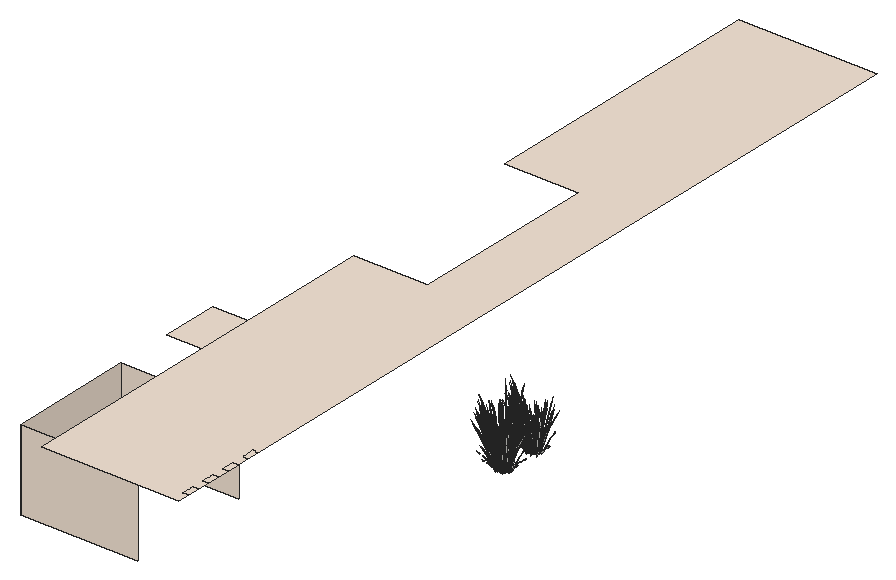
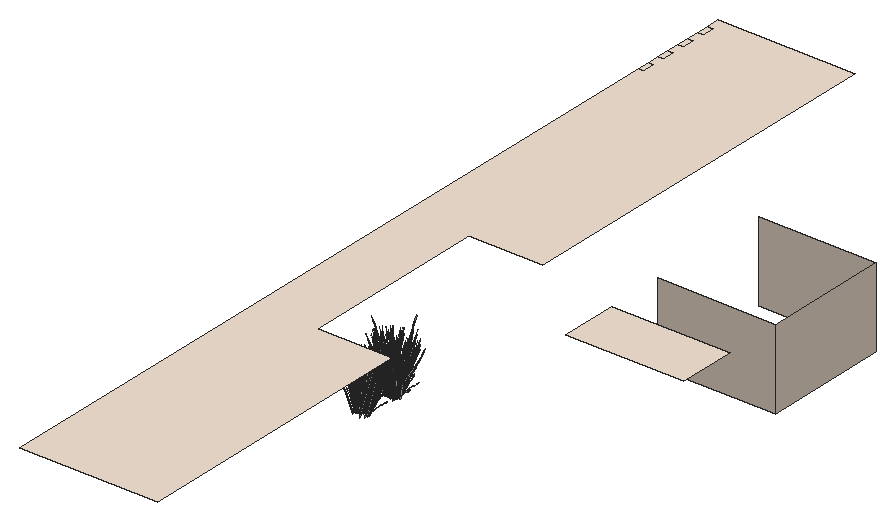
# SketchUp Ruby script. Lengths in inches.
U = 1.inch
M = Sketchup.active_model
def pt(a) = Geom::Point3d.new(a.map { |v| v * U })
def face(e, loops, mat)
  f = e.add_face(loops[0].map { |a| pt(a) })
  loops[1..].each { |l| e.add_face(l.map { |a| pt(a) }).erase! }
  f.material = f.back_material = mat if mat
  f
end
# faces: each face lists its corners as indices into pts; further lists are holes
def faces(e, pts, list, mat = nil) = list.each { |f| face(e, (f[0].is_a?(Array) ? f : [f]).map { |l| l.map { |i| pts[i] } }, mat) }
# xy, xz, yz: faces in a plane at the given z, y or x. An outline is a flat list of corners, or four numbers for a rectangle; further outlines are holes
def ring(l) = l.size == 4 ? [[l[0], l[1]], [l[2], l[1]], [l[2], l[3]], [l[0], l[3]]] : l.each_slice(2).to_a
def flat(e, list, mat, &to3) = list.each { |f| face(e, (f[0].is_a?(Array) ? f : [f]).map { |l| ring(l).map { |u, v| to3.(u, v) } }, mat) }
def xy(e, z, list, mat = nil) = flat(e, list, mat) { |x, y| [x, y, z] }
def xz(e, y, list, mat = nil) = flat(e, list, mat) { |x, z| [x, y, z] }
def yz(e, x, list, mat = nil) = flat(e, list, mat) { |y, z| [x, y, z] }
def lines(e, pts, list) = list.each { |a, b| e.add_line(pt(pts[a]), pt(pts[b])) }
# prism: a flat outline (further loops are holes) pulled along v
def prism(e, loops, v, mat = nil)
  f = face(e, loops, mat); d = Geom::Vector3d.new(v.map { |x| x * U })
  f.pushpull(f.normal.samedirection?(d) ? d.length : -d.length)
end
def box(e, o, s, mat = nil) = prism(e, [[o, [o[0] + s[0], o[1], o[2]], [o[0] + s[0], o[1] + s[1], o[2]], [o[0], o[1] + s[1], o[2]]]], [0, 0, s[2]], mat)
def at(x, y, z, deg = 0) = Geom::Transformation.translation(pt([x, y, z])) * Geom::Transformation.rotation(ORIGIN, Z_AXIS, deg.degrees)
def axes(o, x, y, z) = Geom::Transformation.new([*x, 0, *y, 0, *z, 0, *pt(o).to_a, 1])
def part(name) = M.definitions.add(name)
# library, detail: a bought-in or finely detailed component or shape, given as its bounding box
def library(name, o, s) = part(name).tap { |d| box(d.entities, o, s) }
def detail(e, o, s) = box(e.add_group.entities, o, s)
def put(e, d, t, mat = nil) = e.add_instance(d, t).tap { |i| i.material = mat if mat }
def group(e, t, mat = nil) = e.add_group.tap { |g| g.transformation = t; g.material = mat if mat }.entities
root = M.entities
M.materials.add("C01_Vanilla_Cream").color = [244, 228, 212]
M.materials.add("LightPink_Translucent").color = [144, 107, 117]
M.materials["LightPink_Translucent"].alpha = 0.75
c1 = part("blade")
p = [[2.15,0.21,22],[0,0.17,0],[0.09,0.45,0],[2.18,0.31,22],[2.29,0.31,22],[0.38,0.45,0],
  [2.48,0.24,33],[2.49,0.24,33],[2.48,0.22,33]]
faces(c1.entities,p,[[0,1,2,3],[4,5,2,3],[6,3,4,7],[8,0,3,6]])
c2 = part("seeds")
p = [[0.3,-0.1,1.38],[-0.01,-0.03,1.59],[-0.01,-0.03,0.03],[0.14,-0.07,-0.07],[0.29,-0.03,3],[0.15,0.01,3.11]]
faces(c2.entities,p,[[0,1,2,3],[1,0,4,5]],"LightPink_Translucent")
c3 = part("blade with seeds")
put(c3.entities,c1,at(0,0,0))
put(c3.entities,c2,axes([2.4,0.25,30.99],[1.5799,-0.05474,1.17369],[-0.12525,1.92788,0.29478],[-0.07173,-0.02425,1.56792]))
xy(root,393,[[226.53,171,288,201]],"C01_Vanilla_Cream")
xy(root,432,[[288,12,288,216,326.85,216,326.85,314.71,288,314.71,288,468,360,468,360,63.65,357,63.65,357,57.2,360,57.2,360,50.74,357,50.74,357,44.28,360,44.28,360,37.83,357,37.83,357,31.37,360,31.37,360,24.91,357,24.91,357,18.46,360,18.46,360,12],[357,18.46,360,24.91],[357,31.37,360,37.83],[357,44.28,360,50.74],[357,57.2,360,63.65]],"C01_Vanilla_Cream")
xz(root,75,[[226.53,351,288,393]],"C01_Vanilla_Cream")
xz(root,141,[[226.53,351,288,393]],"C01_Vanilla_Cream")
yz(root,226.53,[[75,351,141,393]],"C01_Vanilla_Cream")
put(root,c3,axes([356.25,225,350.91],[0.12726,0.15818,1.28532],[-0.58807,0.13317,0.10393],[-0.13291,-0.24832,0.54946]))
put(root,c3,axes([357.22,223.95,351.54],[-0.08515,-0.06907,1.31208],[-0.56828,0.04379,-0.2075],[-0.0907,-0.16522,0.10523]))
put(root,c3,axes([357.82,225.12,351.74],[-0.26572,-0.40059,-0.53284],[0.54698,-0.22325,0.0643],[-0.06214,-0.19355,0.75375]))
put(root,c3,axes([358.92,225.51,351.74],[0.01449,-0.45571,-0.53284],[0.61002,0.03061,0.0643],[0.06438,-0.19306,0.75375]))
put(root,c3,axes([359.77,224.8,351.54],[-0.00537,-0.09805,1.31208],[-0.45391,-0.28338,-0.2075],[0.07018,-0.17178,0.10523]))
put(root,c3,axes([357.87,224.78,351.39],[0.16784,-0.37886,-0.2656],[0.48968,0.1105,0.3429],[-0.0449,-0.15254,0.65611]))
put(root,c3,axes([358.24,225.28,350.91],[-0.10366,0.16934,1.28532],[-0.43488,-0.35044,0.10393],[0.19618,-0.21841,0.54946]))
put(root,c3,axes([359.65,224.44,351.53],[-0.05654,0.03763,1.33037],[-0.55396,-0.12696,-0.12571],[-0.02005,-0.16422,0.23543]))
put(root,c3,axes([357.62,225.04,351.51],[-0.54728,-0.1235,-0.38324],[0.18759,-0.42344,-0.29685],[-0.05018,-0.17048,0.7333]))
put(root,c3,axes([358.8,225.36,351.51],[-0.39855,-0.33102,-0.38324],[0.42102,-0.2899,-0.29685],[0.06064,-0.16819,0.7333]))
put(root,c3,axes([356.64,223.72,351.53],[-0.01039,0.05905,1.33037],[-0.51226,0.21431,-0.12571],[-0.15074,-0.10955,0.23543]))
put(root,c3,axes([356.52,224.77,351.82],[0.62019,-0.12663,0.40322],[0.10763,0.49673,0.33247],[-0.14586,-0.1464,0.83437]))
put(root,c3,axes([357.93,224.86,351.55],[0.54859,0.1288,0.36002],[-0.18759,0.42344,0.29685],[-0.03297,-0.16652,0.74497]))
put(root,c3,axes([358.08,225.02,351.78],[-0.54481,0.22937,-0.0912],[-0.26773,-0.4071,-0.50621],[-0.07188,-0.17155,0.76918]))
put(root,c3,axes([359.22,225.53,351.78],[-0.61188,-0.02441,-0.0912],[0.01672,-0.46217,-0.50621],[0.0425,-0.178,0.76918]))
put(root,c3,axes([359.17,225.23,351.39],[0.3767,-0.25939,-0.2656],[0.3566,0.29618,0.3429],[0.05426,-0.15048,0.65611]))
put(root,c3,axes([358.07,224.83,351.55],[0.41024,-0.16744,0.04823],[0.2008,0.30532,0.37966],[-0.03962,-0.13459,0.57892]))
put(root,c3,axes([356.62,225.23,351.74],[-0.47473,-0.23813,-0.53284],[0.33738,-0.41728,0.0643],[-0.172,-0.14218,0.75375]))
put(root,c3,axes([356.45,224.91,351.39],[-0.08599,-0.39682,-0.2656],[0.49155,-0.10478,0.3429],[-0.13203,-0.11372,0.65611]))
put(root,c3,axes([356.67,224.88,351.55],[0.25304,-0.31296,0.04823],[0.36033,0.18221,0.37966],[-0.11649,-0.10034,0.57892]))
put(root,c3,axes([355.4,225.49,350.91],[0.2068,0.08488,1.28532],[-0.42797,0.35609,0.10393],[-0.26673,-0.16064,0.54946]))
put(root,c3,axes([357.92,225.17,351.79],[-0.16784,0.37886,0.2656],[-0.48968,-0.1105,-0.3429],[-0.0449,-0.15254,0.65611]))
put(root,c3,axes([356.4,225.24,351.51],[-0.54938,0.11711,-0.38324],[-0.0961,-0.44351,-0.29685],[-0.14756,-0.1271,0.7333]))
put(root,c3,axes([359.17,225.33,351.55],[0.39645,0.33614,0.36002],[-0.42102,0.2899,0.29685],[0.07313,-0.15771,0.74497]))
put(root,c3,axes([356.78,224.85,352.07],[-0.37157,0.4723,-0.10215],[-0.5381,-0.2721,-0.56695],[-0.18705,-0.13344,0.86148]))
put(root,c3,axes([359.32,225.37,351.55],[0.45752,0.02296,0.04823],[-0.01254,0.34663,0.37966],[0.04787,-0.13278,0.57892]))
put(root,c3,axes([358.98,225.6,351.79],[-0.3767,0.25939,0.2656],[-0.3566,-0.29618,-0.3429],[0.05426,-0.15048,0.65611]))
put(root,c3,axes([359.64,226.3,351.74],[0.29081,-0.38873,-0.53284],[0.5096,0.27626,0.0643],[0.17364,-0.14084,0.75375]))
put(root,c3,axes([359.625,226.12,351.51],[-0.14302,-0.44985,-0.38324],[0.54163,-0.07869,-0.29685],[0.15522,-0.12083,0.7333]))
put(root,c3,axes([355.36,224.71,351.54],[-0.11979,-0.00348,1.31208],[-0.38137,0.34775,-0.2075],[-0.20349,-0.07106,0.10523]))
put(root,c3,axes([359.88,226.44,351.78],[-0.515,-0.27165,-0.0912],[0.2967,-0.3934,-0.50621],[0.1455,-0.13675,0.76918]))
put(root,c3,axes([357.75,227.92,350.49],[0.48111,0.19866,1.13446],[-0.47133,0.42798,0.44862],[-0.21112,-0.25366,0.95105]))
put(root,c3,axes([356.75,225.24,351.79],[0.08599,0.39682,0.2656],[-0.49155,0.10478,-0.3429],[-0.13203,-0.11372,0.65611]))
put(root,c3,axes([355.27,225.5,351.82],[0.45978,-0.36358,0.40322],[0.39653,0.38611,0.33247],[-0.21571,-0.06707,0.83437]))
put(root,c3,axes([361.15,226.32,351.53],[-0.07272,-0.00374,1.33037],[-0.30197,-0.40092,-0.12571],[0.12127,-0.13182,0.23543]))
put(root,c3,axes([360.03,226.17,351.39],[0.48462,-0.07041,-0.2656],[0.12797,0.4025,0.3429],[0.13888,-0.10811,0.65611]))
put(root,c3,axes([355.48,225.49,351.55],[0.02803,-0.37463,0.04823],[0.42332,0.01027,0.37966],[-0.16216,-0.0392,0.57892]))
put(root,c3,axes([355.32,225.61,351.39],[-0.31678,-0.30846,-0.2656],[0.36171,-0.29199,0.3429],[-0.18378,-0.04443,0.65611]))
put(root,c3,axes([359.63,226.4,351.79],[-0.48462,0.07041,0.2656],[-0.12797,-0.4025,-0.3429],[0.13888,-0.10811,0.65611]))
put(root,c3,axes([355.65,225.82,351.74],[-0.55654,-0.01186,-0.53284],[0.03738,-0.49951,0.0643],[-0.23578,-0.05271,0.75375]))
put(root,c3,axes([360.07,226.34,351.55],[0.3822,0.20719,0.04823],[-0.22252,0.29505,0.37966],[0.12254,-0.09539,0.57892]))
put(root,c3,axes([359.96,226.25,351.55],[0.13808,0.45342,0.36002],[-0.54163,0.07869,0.29685],[0.15963,-0.10664,0.74497]))
put(root,c3,axes([361.42,226.8,351.54],[0.07726,-0.07504,1.31208],[-0.09888,-0.46032,-0.2075],[0.19384,-0.08728,0.10523]))
put(root,c3,axes([354.9,225,351.53],[0.04127,0.04917,1.33037],[-0.19898,0.44196,-0.12571],[-0.20151,0.0032,0.23543]))
put(root,c3,axes([355.47,225.92,351.51],[-0.40426,0.32635,-0.38324],[-0.35404,-0.34474,-0.29685],[-0.2054,-0.04965,0.7333]))
put(root,c3,axes([355.77,225.77,351.79],[0.31678,0.30846,0.2656],[-0.36171,0.29199,-0.3429],[-0.18378,-0.04443,0.65611]))
put(root,c3,axes([355.68,225.58,351.78],[-0.02981,0.50103,-0.0912],[-0.56442,-0.01369,-0.50621],[-0.21738,-0.0348,0.76918]))
put(root,c3,axes([359.9,227.5,351.78],[-0.28012,-0.44611,-0.0912],[0.49717,-0.21923,-0.50621],[0.20951,-0.05886,0.76918]))
put(root,c3,axes([359.88,227.12,351.51],[0.15083,-0.44814,-0.38324],[0.51712,0.15361,-0.29685],[0.2082,-0.04109,0.7333]))
put(root,c3,axes([354.96,226.27,350.91],[0.23093,-0.01116,1.28532],[-0.15319,0.4836,0.10393],[-0.32909,-0.02991,0.54946]))
put(root,c3,axes([359.78,227.28,351.74],[0.48922,-0.21758,-0.53284],[0.27264,0.44789,0.0643],[0.23638,-0.05088,0.75375]))
put(root,c3,axes([359.71,227.37,351.79],[-0.46269,-0.13744,0.2656],[0.13495,-0.40096,-0.3429],[0.18628,-0.03677,0.65611]))
put(root,c3,axes([354.86,226.63,351.55],[0.15729,-0.44921,0.36002],[0.51712,0.15361,0.29685],[-0.20336,0.027,0.74497]))
put(root,c3,axes([354.83,226.51,351.55],[-0.20448,-0.33592,0.04823],[0.37288,-0.16442,0.37966],[-0.16437,0.03244,0.57892]))
put(root,c3,axes([360.2,227.32,351.39],[0.46269,0.13744,-0.2656],[-0.13495,0.40096,0.3429],[0.18628,-0.03677,0.65611]))
put(root,c3,axes([354.76,226.68,351.39],[-0.46269,-0.13744,-0.2656],[0.13495,-0.40096,0.3429],[-0.18628,0.03677,0.65611]))
put(root,c3,axes([358.93,226.83,350.91],[-0.23093,0.01116,1.28532],[0.15319,-0.4836,0.10393],[0.32909,0.02991,0.54946]))
put(root,c3,axes([360.13,227.49,351.55],[0.20448,0.33592,0.04823],[-0.37288,0.16442,0.37966],[0.16437,-0.03244,0.57892]))
put(root,c3,axes([360.09,227.37,351.55],[-0.15729,0.44921,0.36002],[-0.51712,-0.15361,0.29685],[0.20336,-0.027,0.74497]))
put(root,c3,axes([355.24,226.64,351.79],[0.46269,0.13744,0.2656],[-0.13495,0.40096,-0.3429],[-0.18628,0.03677,0.65611]))
put(root,c3,axes([356.17,226.62,350.51],[0.15825,-0.07127,1.32798],[0.05457,0.4976,0.10393],[-0.34278,0.06603,0.47463]))
put(root,c3,axes([361.02,228.83,351.53],[-0.05034,-0.04313,1.33037],[0.11012,-0.46232,-0.12571],[0.1983,-0.02954,0.23543]))
put(root,c3,axes([354.47,226.95,351.54],[-0.09091,0.06396,1.31208],[0.00773,0.46734,-0.2075],[-0.20839,0.06078,0.10523]))
put(root,c3,axes([355.07,226.89,351.51],[-0.15083,0.44814,-0.38324],[-0.51712,-0.15361,-0.29685],[-0.2082,0.04109,0.7333]))
put(root,c3,axes([355.05,226.5,351.78],[0.28012,0.44611,-0.0912],[-0.49717,0.21923,-0.50621],[-0.20951,0.05886,0.76918]))
put(root,c3,axes([360.58,228.44,350.95],[-0.10656,-0.41414,-0.02619],[0.50364,-0.09521,-0.11874],[0.10517,0.02626,0.39164]))
put(root,c3,axes([359.27,228.43,351.78],[0.02981,-0.50103,-0.0912],[0.56442,0.01369,-0.50621],[0.21738,0.0348,0.76918]))
put(root,c3,axes([359.1875,228.23,351.79],[-0.31678,-0.30846,0.2656],[0.36171,-0.29199,-0.3429],[0.18378,0.04443,0.65611]))
put(root,c3,axes([359.76,228.125,351.54],[0.11943,-0.00833,1.31208],[0.32759,-0.38275,-0.2075],[0.21244,0.05052,0.10523]))
put(root,c3,axes([354.99,227.75,351.55],[-0.13808,-0.45342,0.36002],[0.54163,-0.07869,0.29685],[-0.15963,0.10664,0.74497]))
put(root,c3,axes([354.88,227.66,351.55],[-0.3822,-0.20719,0.04823],[0.22252,-0.29505,0.37966],[-0.12254,0.09539,0.57892]))
put(root,c3,axes([355.06,227.12,350.91],[0.19317,-0.10421,1.28532],[0.16263,0.48153,0.10393],[-0.30326,0.10883,0.54946]))
put(root,c3,axes([359.3,228.1875,351.74],[0.55654,0.01186,-0.53284],[-0.03738,0.49951,0.0643],[0.23578,0.05271,0.75375]))
put(root,c3,axes([355.32,227.6,351.79],[0.48462,-0.07041,0.2656],[0.12797,0.4025,-0.3429],[-0.13888,0.10811,0.65611]))
put(root,c3,axes([353.46,227.42,351.53],[0.07105,0.01321,1.33037],[0.2198,0.43529,-0.12571],[-0.14545,0.11425,0.23543]))
put(root,c3,axes([359.64,228.39,351.39],[0.31678,0.30846,-0.2656],[-0.36171,0.29199,0.3429],[0.18378,0.04443,0.65611]))
put(root,c3,axes([359.47,228.51,351.55],[-0.02803,0.37463,0.04823],[-0.42332,-0.01027,0.37966],[0.16216,0.0392,0.57892]))
put(root,c3,axes([354.93,227.84,351.39],[-0.48462,0.07041,-0.2656],[-0.12797,-0.4025,0.3429],[-0.13888,0.10811,0.65611]))
put(root,c3,axes([359.51,228.39,351.55],[-0.41051,0.32462,0.36002],[-0.35404,-0.34474,0.29685],[0.1926,0.05988,0.74497]))
put(root,c3,axes([354.22,228.74,352.23],[0.49129,0.13151,-0.04866],[-0.15113,0.40475,-0.22062],[-0.08035,0.06145,0.72768]))
put(root,c3,axes([358.21,228.77,351.79],[-0.08599,-0.39682,0.2656],[0.49155,-0.10478,-0.3429],[0.13203,0.11372,0.65611]))
put(root,c3,axes([358.5,227.6,350.91],[-0.2068,-0.08488,1.28532],[0.42797,-0.35609,0.10393],[0.26673,0.16064,0.54946]))
put(root,c3,axes([358.54,226.48,351.36],[-0.48108,-0.25598,1.03712],[0.50798,-0.39855,0.44749],[0.15521,0.24018,1.00248]))
put(root,c3,axes([355.07,227.5625,351.78],[0.515,0.27165,-0.0912],[-0.2967,0.3934,-0.50621],[-0.1455,0.13675,0.76918]))
put(root,c3,axes([358.16,228.97,351.78],[0.33176,-0.4217,-0.0912],[0.48044,0.24295,-0.50621],[0.16701,0.11914,0.76918]))
put(root,c3,axes([355.76,227.44,350.91],[0.13906,-0.15138,1.28532],[0.35111,0.40859,0.10393],[-0.24082,0.18608,0.54946]))
put(root,c3,axes([355.33,227.89,351.51],[0.14302,0.44985,-0.38324],[-0.54163,0.07869,-0.29685],[-0.15522,0.12083,0.7333]))
put(root,c3,axes([355.98,228.4,351.79],[0.3767,-0.25939,0.2656],[0.3566,0.29618,-0.3429],[-0.05426,0.15048,0.65611]))
put(root,c3,axes([357.73,229.32,351.53],[0.00165,-0.05965,1.33037],[0.47711,-0.26315,-0.12571],[0.16572,0.09393,0.23543]))
put(root,c3,axes([358.5,226.97,350.13],[-0.01521,-0.46386,1.05954],[0.68831,0.12024,0.44862],[-0.1628,0.25382,1.00012]))
put(root,c3,axes([355.63,228.64,351.55],[-0.45752,-0.02296,0.04823],[0.01254,-0.34663,0.37966],[-0.04787,0.13278,0.57892]))
put(root,c3,axes([355.78,228.67,351.55],[-0.39645,-0.33614,0.36002],[0.42102,-0.2899,0.29685],[-0.07313,0.15771,0.74497]))
put(root,c3,axes([358.56,228.76,351.51],[0.54938,-0.11711,-0.38324],[0.0961,0.44351,-0.29685],[0.14756,0.1271,0.7333]))
put(root,c3,axes([357.03,228.83,351.79],[0.16784,-0.37886,0.2656],[0.48968,0.1105,-0.3429],[0.0449,0.15254,0.65611]))
put(root,c3,axes([358.29,229.125,351.55],[-0.25304,0.31296,0.04823],[-0.36033,-0.18221,0.37966],[0.11649,0.10034,0.57892]))
put(root,c3,axes([357.69,230.18,352.23],[0.38473,-0.28263,-0.04866],[0.35252,0.30954,-0.22062],[0.02482,0.08771,0.72768]))
put(root,c3,axes([358.39,229.04,351.55],[-0.55374,0.11306,0.36002],[-0.0961,-0.44351,0.29685],[0.13023,0.13071,0.74497]))
put(root,c3,axes([355.66,227.82,350.91],[0.10366,-0.16934,1.28532],[0.43488,0.35044,0.10393],[-0.19618,0.21841,0.54946]))
put(root,c3,axes([356.88,229.17,351.55],[-0.41024,0.16744,0.04823],[-0.2008,-0.30532,0.37966],[0.03962,0.13459,0.57892]))
put(root,c3,axes([355.78,228.77,351.39],[-0.3767,0.25939,-0.2656],[-0.3566,-0.29618,0.3429],[-0.05426,0.15048,0.65611]))
put(root,c3,axes([354.48,228.69,351.54],[-0.01384,0.09749,1.31208],[0.39274,0.33916,-0.2075],[-0.10282,0.16039,0.10523]))
put(root,c3,axes([355.74,228.47,352.05],[0.61188,0.02441,-0.10123],[-0.01672,0.46217,-0.56189],[-0.0425,0.178,0.85379]))
put(root,c3,axes([356.87,228.99,351.78],[0.54481,-0.22937,-0.0912],[0.26773,0.4071,-0.50621],[0.07188,0.17155,0.76918]))
put(root,c3,axes([357.03,229.14,351.8],[-0.54859,-0.1288,0.39962],[0.18759,-0.42344,0.32951],[0.03297,0.16652,0.82692]))
put(root,c3,axes([356.15,228.65,351.75],[0.39855,0.33102,-0.4254],[-0.42102,0.2899,-0.32951],[-0.06064,0.16819,0.81396]))
put(root,c3,axes([357.34,228.97,351.51],[0.54728,0.1235,-0.38324],[-0.18759,0.42344,-0.29685],[0.05018,0.17048,0.7333]))
put(root,c3,axes([357.65,228.1,350.91],[-0.12726,-0.15818,1.28532],[0.58807,-0.13317,0.10393],[0.13291,0.24832,0.54946]))
put(root,c3,axes([357.09,229.23,351.39],[-0.16784,0.37886,-0.2656],[-0.48968,-0.1105,0.3429],[0.0449,0.15254,0.65611]))
put(root,c3,axes([356.03,228.5,352],[-0.01449,0.45571,-0.59145],[-0.61002,-0.03061,0.07138],[-0.06438,0.19306,0.83667]))
put(root,c3,axes([354.4375,229.69,351.53],[0.06316,-0.02974,1.33037],[0.52204,0.19785,-0.12571],[-0.01227,0.16473,0.23543]))
put(root,c3,axes([356.61,228.17,350.91],[-0.01363,-0.18909,1.28532],[0.5906,0.12544,0.10393],[-0.03653,0.26947,0.54946]))
put(root,c3,axes([357.14,228.89,351.74],[0.26572,0.40059,-0.53284],[-0.54698,0.22325,0.0643],[0.06214,0.19355,0.75375]))
put(root,c3,axes([356.74,229.9,351.54],[0.07057,0.07933,1.31208],[0.56952,0.03117,-0.2075],[0.05727,0.17496,0.10523]))
put(root,c3,axes([355.83,229.14,350.52],[0.01223,-0.25433,1.15759],[0.55017,0.13434,0.15997],[-0.04767,0.27105,0.54661]))
put(root,c3,axes([356.25,245.57,350.91],[0.12726,0.15818,1.28532],[-0.58807,0.13317,0.10393],[-0.13291,-0.24832,0.54946]))
put(root,c3,axes([357.22,244.52,351.54],[-0.08515,-0.06907,1.31208],[-0.56828,0.04379,-0.2075],[-0.0907,-0.16522,0.10523]))
put(root,c3,axes([357.82,245.69,351.74],[-0.26572,-0.40059,-0.53284],[0.54698,-0.22325,0.0643],[-0.06214,-0.19355,0.75375]))
put(root,c3,axes([358.92,246.08,351.74],[0.01449,-0.45571,-0.53284],[0.61002,0.03061,0.0643],[0.06438,-0.19306,0.75375]))
put(root,c3,axes([359.77,245.37,351.54],[-0.00537,-0.09805,1.31208],[-0.45391,-0.28338,-0.2075],[0.07018,-0.17178,0.10523]))
put(root,c3,axes([357.87,245.35,351.39],[0.16784,-0.37886,-0.2656],[0.48968,0.1105,0.3429],[-0.0449,-0.15254,0.65611]))
put(root,c3,axes([358.24,245.85,350.91],[-0.10366,0.16934,1.28532],[-0.43488,-0.35044,0.10393],[0.19618,-0.21841,0.54946]))
put(root,c3,axes([359.65,245.02,351.53],[-0.05654,0.03763,1.33037],[-0.55396,-0.12696,-0.12571],[-0.02005,-0.16422,0.23543]))
put(root,c3,axes([357.62,245.61,351.51],[-0.54728,-0.1235,-0.38324],[0.18759,-0.42344,-0.29685],[-0.05018,-0.17048,0.7333]))
put(root,c3,axes([357.95,244.55,350.07],[0.07142,0.28728,0.86145],[-0.3962,-0.15911,0.63294],[0.04263,-0.1471,0.18974]))
put(root,c3,axes([358.8,245.93,351.51],[-0.39855,-0.33102,-0.38324],[0.42102,-0.2899,-0.29685],[0.06064,-0.16819,0.7333]))
put(root,c3,axes([356.64,244.3,351.53],[-0.01039,0.05905,1.33037],[-0.51226,0.21431,-0.12571],[-0.15074,-0.10955,0.23543]))
put(root,c3,axes([356.52,245.34,351.82],[0.62019,-0.12663,0.40322],[0.10763,0.49673,0.33247],[-0.14586,-0.1464,0.83437]))
put(root,c3,axes([357.93,245.4375,351.55],[0.54859,0.1288,0.36002],[-0.18759,0.42344,0.29685],[-0.03297,-0.16652,0.74497]))
put(root,c3,axes([358.08,245.59,351.78],[-0.54481,0.22937,-0.0912],[-0.26773,-0.4071,-0.50621],[-0.07188,-0.17155,0.76918]))
put(root,c3,axes([359.22,246.1,351.78],[-0.61188,-0.02441,-0.0912],[0.01672,-0.46217,-0.50621],[0.0425,-0.178,0.76918]))
put(root,c3,axes([359.17,245.81,351.39],[0.3767,-0.25939,-0.2656],[0.3566,0.29618,0.3429],[0.05426,-0.15048,0.65611]))
put(root,c3,axes([355.92,244.89,350.07],[0.29042,0.17147,0.86145],[-0.42295,0.10307,0.63294],[-0.0905,-0.13178,0.18974]))
put(root,c3,axes([358.07,245.41,351.55],[0.41024,-0.16744,0.04823],[0.2008,0.30532,0.37966],[-0.03962,-0.13459,0.57892]))
put(root,c3,axes([356.62,245.8,351.74],[-0.47473,-0.23813,-0.53284],[0.33738,-0.41728,0.0643],[-0.172,-0.14218,0.75375]))
put(root,c3,axes([356.45,245.49,351.39],[-0.08599,-0.39682,-0.2656],[0.49155,-0.10478,0.3429],[-0.13203,-0.11372,0.65611]))
put(root,c3,axes([356.67,245.45,351.55],[0.25304,-0.31296,0.04823],[0.36033,0.18221,0.37966],[-0.11649,-0.10034,0.57892]))
put(root,c3,axes([355.4,246.07,350.91],[0.2068,0.08488,1.28532],[-0.42797,0.35609,0.10393],[-0.26673,-0.16064,0.54946]))
put(root,c3,axes([357.92,245.75,351.79],[-0.16784,0.37886,0.2656],[-0.48968,-0.1105,-0.3429],[-0.0449,-0.15254,0.65611]))
put(root,c3,axes([356.4,245.82,351.51],[-0.54938,0.11711,-0.38324],[-0.0961,-0.44351,-0.29685],[-0.14756,-0.1271,0.7333]))
put(root,c3,axes([359.17,245.91,351.55],[0.39645,0.33614,0.36002],[-0.42102,0.2899,0.29685],[0.07313,-0.15771,0.74497]))
put(root,c3,axes([356.78,245.42,352.07],[-0.37157,0.4723,-0.10215],[-0.5381,-0.2721,-0.56695],[-0.18705,-0.13344,0.86148]))
put(root,c3,axes([359.32,245.94,351.55],[0.45752,0.02296,0.04823],[-0.01254,0.34663,0.37966],[0.04787,-0.13278,0.57892]))
put(root,c3,axes([358.98,246.18,351.79],[-0.3767,0.25939,0.2656],[-0.3566,-0.29618,-0.3429],[0.05426,-0.15048,0.65611]))
put(root,c3,axes([359.64,246.875,351.74],[0.29081,-0.38873,-0.53284],[0.5096,0.27626,0.0643],[0.17364,-0.14084,0.75375]))
put(root,c3,axes([359.625,246.69,351.51],[-0.14302,-0.44985,-0.38324],[0.54163,-0.07869,-0.29685],[0.15522,-0.12083,0.7333]))
put(root,c3,axes([355.36,245.28,351.54],[-0.11979,-0.00348,1.31208],[-0.38137,0.34775,-0.2075],[-0.20349,-0.07106,0.10523]))
put(root,c3,axes([359.88,247.01,351.78],[-0.515,-0.27165,-0.0912],[0.2967,-0.3934,-0.50621],[0.1455,-0.13675,0.76918]))
put(root,c3,axes([357.75,248.5,350.49],[0.48111,0.19866,1.13446],[-0.47133,0.42798,0.44862],[-0.21112,-0.25366,0.95105]))
put(root,c3,axes([356.75,245.8125,351.79],[0.08599,0.39682,0.2656],[-0.49155,0.10478,-0.3429],[-0.13203,-0.11372,0.65611]))
put(root,c3,axes([355.27,246.07,351.82],[0.45978,-0.36358,0.40322],[0.39653,0.38611,0.33247],[-0.21571,-0.06707,0.83437]))
put(root,c3,axes([361.15,246.9,351.53],[-0.07272,-0.00374,1.33037],[-0.30197,-0.40092,-0.12571],[0.12127,-0.13182,0.23543]))
put(root,c3,axes([360.29,245.8,350.07],[-0.18544,0.25079,0.86145],[-0.15939,-0.33694,0.63294],[0.15316,-0.08443,0.18974]))
put(root,c3,axes([360.03,246.74,351.39],[0.48462,-0.07041,-0.2656],[0.12797,0.4025,0.3429],[0.13888,-0.10811,0.65611]))
put(root,c3,axes([355.48,246.07,351.55],[0.02803,-0.37463,0.04823],[0.42332,0.01027,0.37966],[-0.16216,-0.0392,0.57892]))
put(root,c3,axes([355.32,246.1875,351.39],[-0.31678,-0.30846,-0.2656],[0.36171,-0.29199,0.3429],[-0.18378,-0.04443,0.65611]))
put(root,c3,axes([359.63,246.98,351.79],[-0.48462,0.07041,0.2656],[-0.12797,-0.4025,-0.3429],[0.13888,-0.10811,0.65611]))
put(root,c3,axes([355.65,246.39,351.74],[-0.55654,-0.01186,-0.53284],[0.03738,-0.49951,0.0643],[-0.23578,-0.05271,0.75375]))
put(root,c3,axes([360.07,246.91,351.55],[0.3822,0.20719,0.04823],[-0.22252,0.29505,0.37966],[0.12254,-0.09539,0.57892]))
put(root,c3,axes([359.96,246.83,351.55],[0.13808,0.45342,0.36002],[-0.54163,0.07869,0.29685],[0.15963,-0.10664,0.74497]))
put(root,c3,axes([361.42,247.375,351.54],[0.07726,-0.07504,1.31208],[-0.09888,-0.46032,-0.2075],[0.19384,-0.08728,0.10523]))
put(root,c3,axes([354.9,245.58,351.53],[0.04127,0.04917,1.33037],[-0.19898,0.44196,-0.12571],[-0.20151,0.0032,0.23543]))
put(root,c3,axes([355.47,246.49,351.51],[-0.40426,0.32635,-0.38324],[-0.35404,-0.34474,-0.29685],[-0.2054,-0.04965,0.7333]))
put(root,c3,axes([355.77,246.35,351.79],[0.31678,0.30846,0.2656],[-0.36171,0.29199,-0.3429],[-0.18378,-0.04443,0.65611]))
put(root,c3,axes([355.68,246.15,351.78],[-0.02981,0.50103,-0.0912],[-0.56442,-0.01369,-0.50621],[-0.21738,-0.0348,0.76918]))
put(root,c3,axes([359.9,248.07,351.78],[-0.28012,-0.44611,-0.0912],[0.49717,-0.21923,-0.50621],[0.20951,-0.05886,0.76918]))
put(root,c3,axes([359.88,247.69,351.51],[0.15083,-0.44814,-0.38324],[0.51712,0.15361,-0.29685],[0.2082,-0.04109,0.7333]))
put(root,c3,axes([354.96,246.84,350.91],[0.23093,-0.01116,1.28532],[-0.15319,0.4836,0.10393],[-0.32909,-0.02991,0.54946]))
put(root,c3,axes([359.78,247.85,351.74],[0.48922,-0.21758,-0.53284],[0.27264,0.44789,0.0643],[0.23638,-0.05088,0.75375]))
put(root,c3,axes([359.71,247.94,351.79],[-0.46269,-0.13744,0.2656],[0.13495,-0.40096,-0.3429],[0.18628,-0.03677,0.65611]))
put(root,c3,axes([354.86,247.21,351.55],[0.15729,-0.44921,0.36002],[0.51712,0.15361,0.29685],[-0.20336,0.027,0.74497]))
put(root,c3,axes([354.83,247.09,351.55],[-0.20448,-0.33592,0.04823],[0.37288,-0.16442,0.37966],[-0.16437,0.03244,0.57892]))
put(root,c3,axes([360.2,247.9,351.39],[0.46269,0.13744,-0.2656],[-0.13495,0.40096,0.3429],[0.18628,-0.03677,0.65611]))
put(root,c3,axes([354.76,247.26,351.39],[-0.46269,-0.13744,-0.2656],[0.13495,-0.40096,0.3429],[-0.18628,0.03677,0.65611]))
put(root,c3,axes([358.93,247.4,350.91],[-0.23093,0.01116,1.28532],[0.15319,-0.4836,0.10393],[0.32909,0.02991,0.54946]))
put(root,c3,axes([360.13,248.0625,351.55],[0.20448,0.33592,0.04823],[-0.37288,0.16442,0.37966],[0.16437,-0.03244,0.57892]))
put(root,c3,axes([360.09,247.95,351.55],[-0.15729,0.44921,0.36002],[-0.51712,-0.15361,0.29685],[0.20336,-0.027,0.74497]))
put(root,c3,axes([355.24,247.21,351.79],[0.46269,0.13744,0.2656],[-0.13495,0.40096,-0.3429],[-0.18628,0.03677,0.65611]))
put(root,c3,axes([356.17,247.19,350.51],[0.15825,-0.07127,1.32798],[0.05457,0.4976,0.10393],[-0.34278,0.06603,0.47463]))
put(root,c3,axes([361.02,249.4,351.53],[-0.05034,-0.04313,1.33037],[0.11012,-0.46232,-0.12571],[0.1983,-0.02954,0.23543]))
